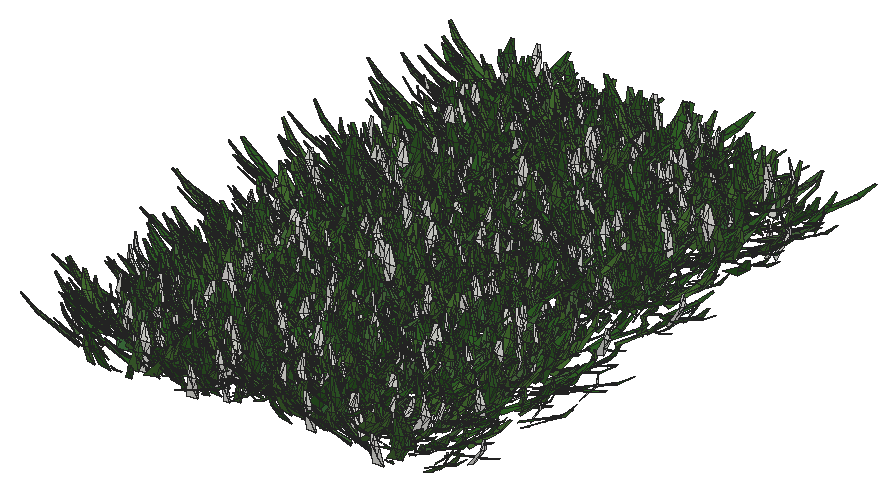
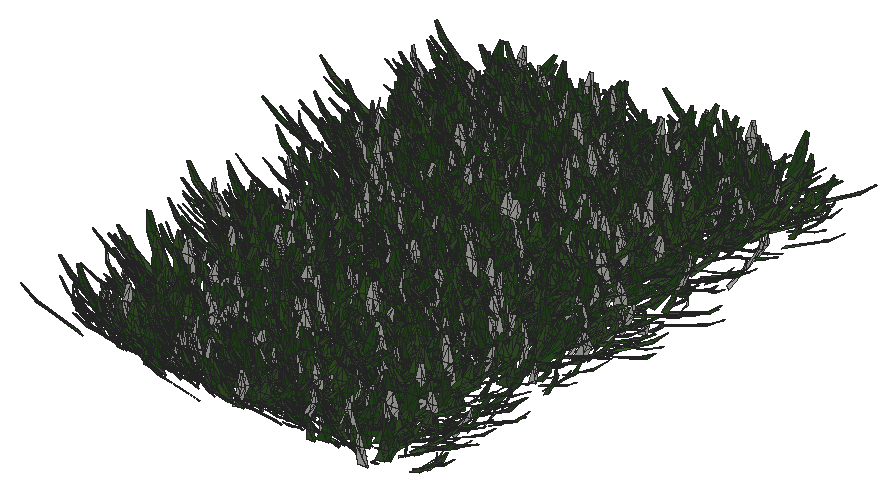
# SketchUp Ruby script. Lengths in inches.
U = 1.inch
M = Sketchup.active_model
def pt(a) = Geom::Point3d.new(a.map { |v| v * U })
def face(e, loops, mat)
  f = e.add_face(loops[0].map { |a| pt(a) })
  loops[1..].each { |l| e.add_face(l.map { |a| pt(a) }).erase! }
  f.material = f.back_material = mat if mat
  f
end
# faces: each face lists its corners as indices into pts; further lists are holes
def faces(e, pts, list, mat = nil) = list.each { |f| face(e, (f[0].is_a?(Array) ? f : [f]).map { |l| l.map { |i| pts[i] } }, mat) }
# xy, xz, yz: faces in a plane at the given z, y or x. An outline is a flat list of corners, or four numbers for a rectangle; further outlines are holes
def ring(l) = l.size == 4 ? [[l[0], l[1]], [l[2], l[1]], [l[2], l[3]], [l[0], l[3]]] : l.each_slice(2).to_a
def flat(e, list, mat, &to3) = list.each { |f| face(e, (f[0].is_a?(Array) ? f : [f]).map { |l| ring(l).map { |u, v| to3.(u, v) } }, mat) }
def xy(e, z, list, mat = nil) = flat(e, list, mat) { |x, y| [x, y, z] }
def xz(e, y, list, mat = nil) = flat(e, list, mat) { |x, z| [x, y, z] }
def yz(e, x, list, mat = nil) = flat(e, list, mat) { |y, z| [x, y, z] }
def lines(e, pts, list) = list.each { |a, b| e.add_line(pt(pts[a]), pt(pts[b])) }
# prism: a flat outline (further loops are holes) pulled along v
def prism(e, loops, v, mat = nil)
  f = face(e, loops, mat); d = Geom::Vector3d.new(v.map { |x| x * U })
  f.pushpull(f.normal.samedirection?(d) ? d.length : -d.length)
end
def box(e, o, s, mat = nil) = prism(e, [[o, [o[0] + s[0], o[1], o[2]], [o[0] + s[0], o[1] + s[1], o[2]], [o[0], o[1] + s[1], o[2]]]], [0, 0, s[2]], mat)
def at(x, y, z, deg = 0) = Geom::Transformation.translation(pt([x, y, z])) * Geom::Transformation.rotation(ORIGIN, Z_AXIS, deg.degrees)
def axes(o, x, y, z) = Geom::Transformation.new([*x, 0, *y, 0, *z, 0, *pt(o).to_a, 1])
def part(name) = M.definitions.add(name)
# library, detail: a bought-in or finely detailed component or shape, given as its bounding box
def library(name, o, s) = part(name).tap { |d| box(d.entities, o, s) }
def detail(e, o, s) = box(e.add_group.entities, o, s)
def put(e, d, t, mat = nil) = e.add_instance(d, t).tap { |i| i.material = mat if mat }
def group(e, t, mat = nil) = e.add_group.tap { |g| g.transformation = t; g.material = mat if mat }.entities
root = M.entities
M.materials.add("Material82").color = [68, 110, 58]
M.materials.add("Material83").color = [48, 90, 38]
M.materials.add("Material84").color = [68, 110, 48]
M.materials.add("Material85").color = [48, 90, 48]
M.materials.add("Material86").color = [58, 110, 58]
M.materials.add("Material87").color = [58, 90, 38]
M.materials.add("Material88").color = [68, 100, 58]
M.materials.add("Material89").color = [48, 100, 38]
c1 = part("grass00")
p = [[-0.6875,0.15,0],[-0.56,0.08,5.52],[-0.04,0.03,2.76],[0.48,-0.02,0],[0.35,-0.02,5.52],[-0.1,-0.14,5.52],
  [-0.12,0.65,8.37],[-0.42,0.65,8.37]]
faces(c1.entities,p,[[0,1,2,3],[3,2,4],[1,5,2],[5,4,2],[1,6,5],[4,5,6],[7,6,1]])
c2 = part("Group16\#1")
put(c2.entities,c1,axes([1.44,-0.61,-0.01],[0.05352,0.12609,0],[-0.10704,0.04543,0.07239],[0.06664,-0.02828,0.11628]),"Material85")
put(c2.entities,c1,axes([0.76,-0.15,-0.01],[0.04676,0.24062,0],[-0.23162,0.04501,0.06642],[0.0652,-0.01267,0.23595]),"Material82")
put(c2.entities,c1,axes([0.79,0.01,-0.01],[-0.00606,0.34651,0],[-0.34381,-0.00602,0.0432],[0.04319,0.00076,0.34386]))
put(c2.entities,c1,axes([1,0.23,-0.01],[-0.07192,0.31144,0],[-0.28722,-0.06632,0.1236],[0.12043,0.02781,0.29478]),"Material84")
put(c2.entities,c1,axes([1.66,0.77,-0.01],[-0.13828,0.29651,0],[-0.21551,-0.1005,0.22471],[0.20365,0.09498,0.23779]),"Material89")
put(c2.entities,c1,axes([0.6875,0.52,-0.01],[-0.18126,0.24051,0],[-0.22746,-0.17142,0.09788],[0.07817,0.05891,0.28481]),"Material84")
put(c2.entities,c1,axes([0.68,0.78,-0.01],[-0.215,0.18688,0],[-0.12385,-0.14248,0.21334],[0.13995,0.16101,0.18878]),"Material82")
put(c2.entities,c1,axes([0.56,1,-0.01],[-0.13756,0.07624,0],[-0.06159,-0.11112,0.0927],[0.04494,0.08108,0.12705]),"Material84")
put(c2.entities,c1,axes([0.2,0.64,-0.01],[-0.23729,0.07254,0],[-0.05711,-0.18681,0.153],[0.04473,0.14632,0.19535]),"Material89")
put(c2.entities,c1,axes([0.0625,0.72,-0.01],[-0.28874,0.02525,0],[-0.02179,-0.24916,0.14647],[0.01276,0.14591,0.25012]),"Material82")
put(c2.entities,c1,axes([-0.08,0.62,-0.01],[-0.34089,-0.04187,0],[0.03255,-0.26504,0.216],[-0.02633,0.21439,0.26703]),"Material89")
put(c2.entities,c1,axes([-0.34,0.98,-0.01],[-0.14314,-0.0493,0],[0.04397,-0.12769,0.06843],[-0.02228,0.0647,0.13505]),"Material89")
put(c2.entities,c1,axes([-0.87,1.45,-0.01],[-0.23488,-0.14114,0],[0.13761,-0.22901,0.06087],[-0.03135,0.05217,0.26717]))
put(c2.entities,c1,axes([-0.72,0.77,-0.01],[-0.14208,-0.13251,0],[0.07209,-0.0773,0.16301],[-0.11118,0.11922,0.1057]),"Material89")
put(c2.entities,c1,axes([-0.62,0.43,-0.01],[-0.14845,-0.21203,0],[0.18654,-0.13061,0.12304],[-0.10079,0.07057,0.22772]),"Material82")
put(c2.entities,c1,axes([-0.68,0.29,-0.01],[-0.13639,-0.32136,0],[0.31723,-0.13464,0.05579],[-0.05136,0.0218,0.34462]),"Material83")
put(c2.entities,c1,axes([-0.64,0.125,-0.01],[-0.0458,-0.23569,0],[0.22124,-0.043,0.08276],[-0.08124,0.01579,0.22538]),"Material86")
put(c2.entities,c1,axes([-1.6,-0.03,-0.01],[0.00576,-0.32897,0],[0.27526,0.00482,0.18018],[-0.18015,-0.00315,0.2753]),"Material84")
put(c2.entities,c1,axes([-1.36,-0.31,-0.01],[0.05718,-0.24765,0],[0.18172,0.04196,0.17267],[-0.16825,-0.03885,0.1865]),"Material89")
put(c2.entities,c1,axes([-1.54,-0.72,-0.01],[0.06537,-0.14017,0],[0.13555,0.06321,0.03939],[-0.0357,-0.01665,0.14956]))
put(c2.entities,c1,axes([-1.19,-0.9,-0.01],[0.09597,-0.12735,0],[0.11214,0.08451,0.07557],[-0.06035,-0.04548,0.14042]),"Material88")
put(c2.entities,c1,axes([-0.47,-0.54,-0.01],[0.11588,-0.10072,0],[0.0618,0.0711,0.12124],[-0.07953,-0.0915,0.0942]))
put(c2.entities,c1,axes([-0.47,-0.84,-0.01],[0.11927,-0.0661,0],[0.06603,0.11913,0.00646],[-0.00313,-0.00565,0.13621]),"Material84")
put(c2.entities,c1,axes([-0.38,-1.24,-0.01],[0.28037,-0.08571,0],[0.0618,0.20215,0.20315],[-0.05939,-0.19428,0.21139]),"Material88")
put(c2.entities,c1,axes([-0.06,-0.66,-0.01],[0.22719,-0.01987,0],[0.01247,0.14255,0.17758],[-0.01547,-0.17691,0.1431]),"Material87")
put(c2.entities,c1,axes([0.11,-0.89,-0.01],[0.14882,0.01828,0],[-0.01058,0.08611,0.12229],[0.01491,-0.12138,0.08676]),"Material85")
put(c2.entities,c1,axes([0.25,-0.72,-0.01],[0.20481,0.07053,0],[-0.06206,0.18022,0.10291],[0.03351,-0.0973,0.1906]),"Material85")
put(c2.entities,c1,axes([0.85,-1.42,-0.01],[0.16481,0.09904,0],[-0.09472,0.15762,0.05616],[0.02893,-0.04814,0.18389]),"Material84")
put(c2.entities,c1,axes([1.01,-1.09,-0.01],[0.21858,0.20385,0],[-0.17495,0.1876,0.15339],[0.10462,-0.11218,0.25652]),"Material89")
put(c2.entities,c1,axes([1.01,-0.71,-0.01],[0.08733,0.12473,0],[-0.06445,0.04512,0.13037],[0.1068,-0.07477,0.07867]),"Material85")
c3 = part("Group15\#1")
put(c3.entities,c2,at(0,0,0))
c4 = part("3darcstudiotree_grass00\#1")
put(c4.entities,c3,at(0,0,0))
put(root,c4,axes([777.29,306.87,-34.17],[1.677,-1.55355,0],[4.28787,0.71988,-0.03539],[0.14144,0.02375,1.51703]))
put(root,c4,axes([777.74,322.0625,-34.17],[-2.71685,-1.17622,0],[2.71806,-0.97644,-0.02128],[0.11147,-0.04005,1.95268]))
put(root,c4,axes([777.99,286.73,-34.17],[-3.01218,-1.1682,0],[2.32929,-0.93411,-0.00764],[0.03903,-0.01565,1.81511]))
put(root,c4,axes([778.03,333.52,-34.17],[0.25601,-1.60576,0],[3.7655,0.09337,-0.00515],[0.03185,0.00079,1.75106]))
put(root,c4,axes([777.02,340.01,-34.17],[3.21046,-0.42194,0],[1.31397,1.55496,-0.01535],[0.02427,0.02872,1.5577]))
put(root,c4,axes([777.04,312.04,-34.17],[-1.88352,1.24088,0],[-3.53635,-0.83485,-0.03562],[-0.13641,-0.0322,1.37892]))
put(root,c4,axes([777.76,283.93,-34.17],[0.35251,-1.39793,0],[3.51175,0.13773,-0.03727],[0.24286,0.00952,1.73202]))
put(root,c4,axes([778.03,289.67,-34.17],[-3.43821,0.20499,0],[-0.69374,-1.80975,-0.03474],[-0.02131,-0.0556,1.42794]))
put(root,c4,axes([777.09,298.68,-34.17],[-0.07716,1.61232,0],[-4.08051,-0.03037,-0.05443],[-0.27918,-0.00208,1.56933]))
put(root,c4,axes([778.64,320.22,-34.17],[1.28288,-1.22527,0],[4.05082,0.65965,-0.04448],[0.2416,0.03934,1.93016]))
put(root,c4,axes([778.91,328.61,-34.17],[-0.2981,-1.54731,0],[4.18924,-0.12553,-0.05563],[0.33136,-0.00993,1.88098]))
put(root,c4,axes([778.75,317.46,-34.17],[-0.54088,1.62044,0],[-3.31155,-0.17191,-0.03263],[-0.19335,-0.01004,1.49628]))
put(root,c4,axes([778.93,315.92,-34.17],[3.70566,-0.42814,0],[1.15173,1.5504,-0.01036],[0.01836,0.02471,1.93559]))
put(root,c4,axes([779.4375,281.24,-34.17],[2.92691,-1.3802,0],[3.11862,1.02859,-0.02296],[0.10607,0.03499,1.8355]))
put(root,c4,axes([780,338.09,-34.17],[-3.14741,0.41412,0],[-1.12782,-1.33315,-0.01591],[-0.02767,-0.03271,1.46774]))
put(root,c4,axes([779.23,335.22,-34.17],[-0.97344,1.33602,0],[-4.5066,-0.51069,-0.06106],[-0.24596,-0.02787,1.47293]))
put(root,c4,axes([779.06,304.44,-34.17],[4.64499,-0.27977,0],[0.53132,1.372,-0.02943],[0.02555,0.06597,1.51666]))
put(root,c4,axes([780.51,302.05,-34.17],[-0.18207,-1.50592,0],[4.09357,-0.07698,-0.05646],[0.28834,-0.00542,1.57058]))
put(root,c4,axes([779.18,291.67,-34.17],[2.47814,1.17598,0],[-3.14029,1.02922,-0.05468],[-0.21842,0.07159,1.58958]))
put(root,c4,axes([779.15,313.96,-34.17],[4.42055,0.62646,0],[-1.4719,1.61538,-0.03831],[-0.06085,0.06679,1.53223]))
put(root,c4,axes([779.68,330.81,-34.17],[4.51641,-0.1704,0],[0.33815,1.39393,-0.00501],[0.00291,0.012,1.62495]))
put(root,c4,axes([779.375,293.85,-34.17],[2.33395,1.59128,0],[-3.69314,0.84246,-0.02506],[-0.12399,0.02828,1.82822]))
put(root,c4,axes([779.96,285.62,-34.17],[3.72841,-0.11021,0],[0.34874,1.83494,-0.00347],[0.00143,0.00753,1.92949]))
put(root,c4,axes([780.95,326.92,-34.17],[-2.15234,1.14546,0],[-3.3995,-0.99347,-0.05517],[-0.2418,-0.07066,1.72999]))
put(root,c4,axes([780.26,300.64,-34.17],[2.3917,1.38211,0],[-2.775,0.74686,-0.01403],[-0.09111,0.02452,1.97952]))
put(root,c4,axes([780.35,309.31,-34.17],[3.05644,0.96272,0],[-2.54771,1.25799,-0.04015],[-0.1144,0.05649,1.39698]))
put(root,c4,axes([780.91,296.33,-34.17],[0.44258,1.4547,0],[-3.4051,0.16112,-0.01784],[-0.12417,0.00588,1.80168]))
put(root,c4,axes([782.55,323.88,-34.17],[-1.45799,-1.43911,0],[3.11235,-0.49041,-0.01431],[0.09188,-0.01448,1.73701]))
put(root,c4,axes([782.7,283.47,-34.17],[-2.77273,1.25915,0],[-2.61353,-0.89509,-0.01448],[-0.05898,-0.0202,1.39954]))
put(root,c4,axes([783.67,285,-34.17],[-3.67224,-0.62774,0],[1.3268,-1.20717,-0.04544],[0.10775,-0.09803,1.4908]))
put(root,c4,axes([783.92,317.6,-34.17],[-4.47177,0.4092,0],[-0.80597,-1.36984,-0.03599],[-0.04373,-0.07433,1.43677]))
put(root,c4,axes([783.3,295.9,-34.17],[-3.07968,1.30519,0],[-3.32937,-1.22181,-0.01383],[-0.04412,-0.01619,1.48532]))
put(root,c4,axes([784.08,339.19,-34.17],[-3.54635,0.32604,0],[-1.06041,-1.79388,-0.06463],[-0.05576,-0.09432,1.33032]))
put(root,c4,axes([782.85,307.32,-34.17],[3.91717,0.58785,0],[-1.40512,1.45623,-0.01203],[-0.02325,0.0241,1.60927]))
put(root,c4,axes([784.71,302.46,-34.17],[-1.04981,-1.26066,0],[3.51989,-0.45588,-0.02104],[0.10484,-0.01358,1.45661]))
put(root,c4,axes([783.97,299.02,-34.17],[3.15172,-0.92963,0],[2.70365,1.42561,-0.02614],[0.06865,0.0362,1.48366]))
put(root,c4,axes([784.75,305.26,-34.17],[-4.56421,0.17831,0],[-0.33265,-1.32435,-0.0174],[-0.0117,-0.04658,1.72585]))
put(root,c4,axes([785.23,330.95,-34.17],[-3.08784,-0.53374,0],[1.78756,-1.6084,-0.00176],[0.00414,-0.00372,1.95594]))
put(root,c4,axes([784.29,291.37,-34.17],[-2.14552,1.35971,0],[-3.80804,-0.93454,-0.04897],[-0.2422,-0.05944,1.9584]))
put(root,c4,axes([783.75,288.08,-34.17],[3.03533,0.518,0],[-1.31858,1.2017,-0.02703],[-0.08286,0.07551,1.9211]))
put(root,c4,axes([785.59,313.28,-34.17],[-2.79081,-0.68685,0],[2.20267,-1.39196,-0.00523],[0.01654,-0.01045,1.86317]))
put(root,c4,axes([785.72,316.69,-34.17],[-3.42781,-0.73376,0],[1.91044,-1.38806,-0.04387],[0.11882,-0.08633,1.70431]))
put(root,c4,axes([785.03,289.42,-34.17],[-3.41152,0.77464,0],[-2.34689,-1.60751,-0.0199],[-0.0471,-0.03226,1.67187]))
put(root,c4,axes([784.04,312.07,-34.17],[1.53269,1.16919,0],[-3.90157,0.79546,-0.03477],[-0.15934,0.03249,1.69826]))
put(root,c4,axes([785.32,300.03,-34.17],[-2.82754,1.11661,0],[-2.90837,-1.14544,-0.05526],[-0.21558,-0.0849,1.69871]))
put(root,c4,axes([785.34,293.44,-34.17],[2.39859,-1.38317,0],[2.89597,0.78107,-0.02882],[0.1286,0.03468,1.42183]))
put(root,c4,axes([785.76,337.85,-34.17],[0.37671,-1.60669,0],[3.58296,0.13066,-0.04487],[0.23434,0.00855,1.41449]))
put(root,c4,axes([786.17,336.35,-34.17],[-4.41181,-0.09171,0],[0.23476,-1.75641,-0.0488],[0.01273,-0.09527,1.65721]))
put(root,c4,axes([786.03,281.67,-34.17],[-3.47293,0.19496,0],[-0.50842,-1.40863,-0.03826],[-0.03299,-0.09141,1.65468]))
put(root,c4,axes([786.59,332.71,-34.17],[-4.2727,-0.29638,0],[0.78575,-1.76178,-0.04722],[0.03378,-0.07573,1.40384]))
put(root,c4,axes([785.25,328.23,-34.17],[-0.9668,1.66725,0],[-3.92404,-0.3539,-0.0233],[-0.11915,-0.01075,1.58282]))
put(root,c4,axes([785.3,309.55,-34.17],[3.78841,0.96012,0],[-2.55963,1.5708,-0.03131],[-0.07104,0.04359,1.48921]))
put(root,c4,axes([785.54,322.55,-34.17],[2.7139,1.45109,0],[-3.63417,1.0571,-0.05484],[-0.17137,0.04985,1.31443]))
put(root,c4,axes([786.1,320.54,-34.17],[3.41186,0.04199,0],[-0.11049,1.39641,-0.01718],[-0.0038,0.04797,1.88076]))
put(root,c4,axes([788.18,299.01,-34.17],[-3.09292,-0.92086,0],[2.57207,-1.3436,-0.01411],[0.04505,-0.02353,1.69584]))
put(root,c4,axes([786.33,326.3125,-34.17],[0.1551,1.54916,0],[-4.73746,0.07377,-0.04149],[-0.18002,0.0028,1.54325]))
put(root,c4,axes([788.36,317.79,-34.17],[0.67498,-1.80639,0],[4.18251,0.24307,-0.00777],[0.03281,0.00191,1.3523]))
put(root,c4,axes([788.52,313.77,-34.17],[-0.75947,-1.30953,0],[4.19896,-0.37875,-0.04627],[0.26037,-0.02349,1.86363]))
put(root,c4,axes([788.5625,300.08,-34.17],[-4.1346,0.13575,0],[-0.2838,-1.34436,-0.02559],[-0.01617,-0.0766,1.95328]))
put(root,c4,axes([789.34,311.39,-34.17],[1.00092,-1.32759,0],[4.42574,0.51896,-0.06029],[0.29852,0.035,1.78762]))
put(root,c4,axes([789.04,332.57,-34.17],[2.10537,-1.23806,0],[3.71835,0.98344,-0.05795],[0.27877,0.07373,1.94389]))
put(root,c4,axes([788.38,287.45,-34.17],[3.79547,0.16316,0],[-0.37027,1.33962,-0.03498],[-0.02197,0.07948,1.48455]))
put(root,c4,axes([789.23,306.96,-34.17],[-3.00276,0.99555,0],[-2.11915,-0.9941,-0.00081],[-0.00373,-0.00175,1.76997]))
put(root,c4,axes([790.35,325.16,-34.17],[-0.04764,-1.42757,0],[4.50476,-0.02338,-0.00745],[0.04284,-0.00022,1.94284]))
put(root,c4,axes([789.05,283.19,-34.17],[0.27257,1.5962,0],[-3.57048,0.09483,-0.04154],[-0.28788,0.00765,1.86323]))
put(root,c4,axes([790.49,320.39,-34.17],[-4.51182,-0.35471,0],[0.87439,-1.72977,-0.01918],[0.02129,-0.04212,1.90358]))
put(root,c4,axes([789.26,327.35,-34.17],[2.9902,-0.77103,0],[1.83544,1.10708,-0.045],[0.13449,0.08112,1.37282]))
put(root,c4,axes([790.54,305.3,-34.17],[0.52861,-1.48035,0],[4.44113,0.24665,-0.00524],[0.03043,0.00169,1.97007]))
put(root,c4,axes([788.83,294.74,-34.17],[1.62026,1.14881,0],[-2.90984,0.63829,-0.00131],[-0.00892,0.00196,1.9458]))
put(root,c4,axes([789.86,285.1875,-34.17],[-3.07094,0.93295,0],[-2.23562,-1.14452,-0.00087],[-0.00325,-0.00166,1.68429]))
put(root,c4,axes([790.9,291.54,-34.17],[-1.32818,-1.26932,0],[4.11875,-0.67029,-0.01762],[0.07227,-0.01176,1.48208]))
put(root,c4,axes([789,289.16,-34.17],[3.48613,0.95688,0],[-2.23612,1.26704,-0.01513],[-0.04219,0.02391,1.43215]))
put(root,c4,axes([790.08,322.25,-34.17],[3.73229,-0.67208,0],[1.78653,1.54305,-0.05401],[0.10032,0.08665,1.44188]))
put(root,c4,axes([791.73,335.35,-34.17],[-3.64932,-0.7532,0],[1.94147,-1.463,-0.05348],[0.14522,-0.10943,1.83786]))
put(root,c4,axes([790.43,309.52,-34.17],[4.39358,-0.14103,0],[0.35283,1.70956,-0.02372],[0.00876,0.04243,1.48337]))
put(root,c4,axes([791.92,336.93,-34.17],[-4.22243,0.41861,0],[-0.86072,-1.35028,-0.03206],[-0.04838,-0.0759,1.63785]))
put(root,c4,axes([790.9375,328.72,-34.17],[2.4549,0.99675,0],[-3.14112,1.20322,-0.03466],[-0.14383,0.05509,1.89896]))
put(root,c4,axes([790.98,315.6,-34.17],[3.48474,0.89145,0],[-2.45497,1.49256,-0.05832],[-0.13986,0.08503,1.48992]))
put(root,c4,axes([791.51,331.39,-34.17],[-0.03901,1.43427,0],[-3.74587,-0.01585,-0.03184],[-0.19446,-0.00082,1.71482]))
put(root,c4,axes([791.9,303.07,-34.17],[-1.95042,1.47202,0],[-4.16072,-0.85742,-0.06253],[-0.2988,-0.06158,1.89715]))
put(root,c4,axes([791.8,296.46,-34.17],[3.54296,-0.10072,0],[0.24357,1.33252,-0.00836],[0.00467,0.02557,1.97523]))
put(root,c4,axes([794,313.82,-34.17],[-3.58618,-0.76762,0],[2.12856,-1.54662,-0.04044],[0.10752,-0.07813,1.86421]))
put(root,c4,axes([792.02,339.32,-34.17],[3.38325,1.26435,0],[-2.73925,1.14001,-0.00751],[-0.0314,0.01307,1.8142]))
put(root,c4,axes([794.27,309.27,-34.17],[-3.71376,-0.4791,0],[1.06109,-1.27925,-0.035],[0.07367,-0.08882,1.73222]))
put(root,c4,axes([794.82,329.42,-34.17],[-3.76687,-0.82913,0],[2.27178,-1.60524,-0.0179],[0.04066,-0.02873,1.62858]))
put(root,c4,axes([793.99,291.75,-34.17],[-3.28554,0.84585,0],[-2.43757,-1.4726,-0.04574],[-0.1384,-0.08361,1.85022]))
put(root,c4,axes([794.73,290.41,-34.17],[0.43132,-1.66774,0],[3.95027,0.1589,-0.00761],[0.04938,0.00199,1.94156]))
put(root,c4,axes([794.99,317.49,-34.17],[-3.03865,-1.23581,0],[2.76731,-1.05827,-0.04714],[0.18592,-0.0711,1.58733]))
put(root,c4,axes([793.58,286.78,-34.17],[4.71636,-0.1967,0],[0.48906,1.82382,-0.02611],[0.01545,0.05763,1.96192]))
put(root,c4,axes([794.67,320.03,-34.17],[-3.07129,1.23004,0],[-2.90171,-1.12685,-0.02428],[-0.07533,-0.02925,1.32917]))
put(root,c4,axes([795.58,294.77,-34.17],[-3.14124,-0.52931,0],[1.80451,-1.66556,-0.04539],[0.09971,-0.09203,1.92461]))
put(root,c4,axes([794.3,338.31,-34.17],[4.37264,-0.16186,0],[0.38997,1.63854,-0.03728],[0.02119,0.08905,1.90298]))
put(root,c4,axes([794.65,332.74,-34.17],[4.22982,-0.69798,0],[1.45654,1.37281,-0.04818],[0.09708,0.0915,1.47658]))
put(root,c4,axes([794.91,331.78,-34.17],[3.5272,-0.10967,0],[0.36977,1.84972,-0.03935],[0.01267,0.0634,1.44542]))
put(root,c4,axes([795.64,324.05,-34.17],[2.22522,-0.98382,0],[3.26699,1.14926,-0.04874],[0.15967,0.05617,1.44038]))
put(root,c4,axes([794.85,298.49,-34.17],[4.40761,-0.00182,0],[0.00468,1.76466,-0.04894],[0.00022,0.08123,1.41164]))
put(root,c4,axes([795.02,339.18,-34.17],[3.37216,0.16863,0],[-0.47809,1.48691,-0.01144],[-0.0086,0.02673,1.7012]))
put(root,c4,axes([796.74,316.68,-34.17],[-3.1255,-0.93872,0],[2.35839,-1.22127,-0.01582],[0.04515,-0.02338,1.37394]))
put(root,c4,axes([795.69,312.24,-34.17],[-2.15998,1.50569,0],[-3.5128,-0.78375,-0.02589],[-0.10439,-0.02329,1.40149]))
put(root,c4,axes([796.18,335.6,-34.17],[2.50422,-1.12718,0],[2.64209,0.91293,-0.00209],[0.0092,0.00318,1.54397]))
put(root,c4,axes([796.33,327.24,-34.17],[-3.79899,1.04858,0],[-2.13311,-1.20197,-0.01309],[-0.05055,-0.02848,1.87779]))
put(root,c4,axes([797,297.02,-34.17],[-0.77442,-1.59147,0],[3.42237,-0.25901,-0.00431],[0.02185,-0.00165,1.34772]))
put(root,c4,axes([797.28,283.77,-34.17],[-1.56215,-1.16443,0],[3.47638,-0.72535,-0.0302],[0.1517,-0.03165,1.67548]))
put(root,c4,axes([797.36,302.51,-34.17],[0.16922,-1.40325,0],[3.56749,0.06691,-0.0123],[0.08099,0.00152,1.7643]))
put(root,c4,axes([796.1875,306.82,-34.17],[3.21803,0.34517,0],[-1.06694,1.54707,-0.02379],[-0.03071,0.04453,1.49895]))
put(root,c4,axes([795.95,300.53,-34.17],[1.18275,1.22871,0],[-4.35683,0.65227,-0.02635],[-0.11985,0.01794,1.69955]))
put(root,c4,axes([797.61,322.41,-34.17],[-4.55654,0.30056,0],[-0.72952,-1.72007,-0.00717],[-0.00538,-0.01268,1.50735]))
put(root,c4,axes([797.1,305.49,-34.17],[2.66801,-0.76193,0],[2.24823,1.2244,-0.04376],[0.15596,0.08494,1.7457]))
put(root,c4,axes([799.2,313.06,-34.17],[-2.4386,-1.43306,0],[3.07254,-0.81318,-0.00883],[0.05033,-0.01332,1.90461]))
put(root,c4,axes([799.57,331.49,-34.17],[-2.69612,-1.17454,0],[3.29179,-1.17522,-0.01753],[0.05781,-0.02064,1.48083]))
put(root,c4,axes([797.53,285.37,-34.17],[-0.169,1.77802,0],[-4.32571,-0.06395,-0.00219],[-0.00941,-0.00014,1.39308]))
put(root,c4,axes([799.77,289.02,-34.17],[-3.83813,-1.06248,0],[2.06139,-1.15817,-0.02484],[0.08815,-0.04953,1.66133]))
put(root,c4,axes([799.46,325.34,-34.17],[-4.08007,0.11151,0],[-0.22831,-1.29918,-0.01842],[-0.00694,-0.03947,1.34789]))
put(root,c4,axes([799.94,283.58,-34.17],[-3.13096,0.65051,0],[-1.62991,-1.22011,-0.01732],[-0.0588,-0.04402,1.90951]))
put(root,c4,axes([801.15,335.92,-34.17],[-1.34356,-1.54381,0],[4.22745,-0.57221,-0.00214],[0.01038,-0.00141,1.72072]))
put(root,c4,axes([799.21,291.125,-34.17],[3.83567,0.80348,0],[-1.71741,1.27513,-0.04207],[-0.13622,0.10114,1.89419]))
put(root,c4,axes([799.63,307.22,-34.17],[2.14752,1.24419,0],[-2.84206,0.76295,-0.02533],[-0.12904,0.03464,1.58831]))
put(root,c4,axes([800.24,329.55,-34.17],[4.00755,-0.76372,0],[1.77132,1.44561,-0.00312],[0.00773,0.00631,1.73901]))
put(root,c4,axes([799.93,300.73,-34.17],[0.92286,1.78615,0],[-4.03148,0.32396,-0.0503],[-0.25163,0.02022,1.57458]))
put(root,c4,axes([800.27,315.79,-34.17],[-1.5079,1.48015,0],[-3.78766,-0.60014,-0.02547],[-0.10708,-0.01697,1.38631]))
put(root,c4,axes([801.32,297.77,-34.17],[0.88426,-1.72062,0],[4.38154,0.35021,-0.041],[0.21175,0.01693,1.76588]))
put(root,c4,axes([800.14,293.66,-34.17],[4.1439,0.48612,0],[-1.21296,1.60815,-0.03162],[-0.038,0.05038,1.3441]))
put(root,c4,axes([800,308.79,-34.17],[2.12924,1.06786,0],[-3.55371,1.10206,-0.01217],[-0.05143,0.01595,1.82194]))
put(root,c4,axes([801.57,284.69,-34.17],[1.5808,-1.43275,0],[3.65536,0.62726,-0.04597],[0.19603,0.03364,1.38947]))
put(root,c4,axes([802.46,288,-34.17],[-4.27451,-0.64112,0],[1.27307,-1.32012,-0.04106],[0.09351,-0.09696,1.71966]))
put(root,c4,axes([802.38,332.92,-34.17],[-3.75297,0.08152,0],[-0.23562,-1.68719,-0.02509],[-0.00578,-0.04142,1.34616]))
put(root,c4,axes([802.375,338.3,-34.17],[-3.08585,0.75112,0],[-1.75968,-1.12437,-0.03387],[-0.09597,-0.06132,1.3548]))
put(root,c4,axes([803.03,323.26,-34.17],[-0.74737,-1.75822,0],[4.00395,-0.2647,-0.02808],[0.1526,-0.01009,1.67665]))
put(root,c4,axes([802.27,304.49,-34.17],[2.37533,-1.57622,0],[3.03149,0.71052,-0.0411],[0.20378,0.04776,1.52451]))
put(root,c4,axes([801.47,317.97,-34.17],[3.22242,0.46316,0],[-1.61234,1.7447,-0.03532],[-0.06153,0.06658,1.79519]))
put(root,c4,axes([801.96,312.34,-34.17],[0.53134,1.4221,0],[-3.42638,0.19911,-0.04131],[-0.21204,0.01232,1.34689]))
put(root,c4,axes([802.45,303.55,-34.17],[3.9417,-1.03975,0],[1.84996,1.09076,-0.03191],[0.12762,0.07525,1.79443]))
put(root,c4,axes([802.83,296.27,-34.17],[3.56947,-0.45549,0],[1.31887,1.60745,-0.01717],[0.02449,0.02985,1.48777]))
put(root,c4,axes([802.91,319.66,-34.17],[0.55525,1.71346,0],[-3.482,0.17549,-0.04145],[-0.30813,0.01553,1.97198]))
put(root,c4,axes([802.66,326.65,-34.17],[3.66484,0.89609,0],[-2.00603,1.27601,-0.03504],[-0.12347,0.07854,1.90819]))
put(root,c4,axes([804.875,289.59,-34.17],[-1.10349,-1.4395,0],[4.41957,-0.52692,-0.03772],[0.14279,-0.01702,1.36861]))
put(root,c4,axes([804.67,319.5,-34.17],[-2.20687,1.14075,0],[-3.09016,-0.92978,-0.05103],[-0.23957,-0.07208,1.72023]))
put(root,c4,axes([805.13,331.53,-34.17],[-3.32366,1.12138,0],[-2.70082,-1.24501,-0.05065],[-0.15287,-0.07047,1.44592]))
put(root,c4,axes([806.22,316.28,-34.17],[-2.7638,-1.30283,0],[3.13183,-1.03331,-0.01878],[0.07913,-0.02611,1.68146]))
put(root,c4,axes([806.45,309,-34.17],[-3.16827,-0.67396,0],[1.62868,-1.19079,-0.04409],[0.1208,-0.08832,1.48398]))
put(root,c4,axes([806.2,317.34,-34.17],[-4.1698,0.79339,0],[-1.666,-1.36181,-0.02532],[-0.06287,-0.05139,1.64221]))
put(root,c4,axes([805.17,337.66,-34.17],[3.81533,0.48086,0],[-1.13696,1.40304,-0.03842],[-0.0798,0.09848,1.90991]))
put(root,c4,axes([805.77,302.06,-34.17],[3.77642,-0.7823,0],[1.66108,1.24712,-0.02304],[0.07142,0.05362,1.78453]))
put(root,c4,axes([807.3,329.27,-34.17],[0.63263,-1.77026,0],[4.09912,0.22783,-0.02402],[0.14113,0.00784,1.84088]))
put(root,c4,axes([807.44,293.54,-34.17],[-4.44839,0.03138,0],[-0.07411,-1.6342,-0.01042],[-0.00109,-0.02408,1.82123]))
put(root,c4,axes([807.43,282.67,-34.17],[-3.4085,0.44598,0],[-1.18576,-1.40948,-0.04681],[-0.08042,-0.0956,1.53984]))
put(root,c4,axes([806.18,292.31,-34.17],[3.54482,0.3991,0],[-1.20365,1.66273,-0.00872],[-0.01104,0.01525,1.51538]))
put(root,c4,axes([806.8125,322.3,-34.17],[-0.28998,1.73456,0],[-3.34694,-0.08702,-0.03816],[-0.29536,-0.00768,1.95014]))
put(root,c4,axes([806.03,287.11,-34.17],[3.41397,1.21641,0],[-2.3032,1.00536,-0.00582],[-0.0237,0.01035,1.56404]))
put(root,c4,axes([806.16,298.54,-34.17],[2.93721,1.2592,0],[-3.10849,1.12772,-0.033],[-0.144,0.05224,1.87715]))
put(root,c4,axes([808.32,300.11,-34.17],[-1.1478,-1.40641,0],[4.093,-0.51953,-0.0477],[0.19511,-0.02477,1.385]))
put(root,c4,axes([808.71,285.97,-34.17],[-2.49924,-1.08664,0],[2.82442,-1.01033,-0.0539],[0.19999,-0.07154,1.43163]))
put(root,c4,axes([807.1,305.5,-34.17],[2.93445,0.88211,0],[-2.13254,1.10335,-0.01463],[-0.05848,0.03025,1.73802]))
put(root,c4,axes([807.22,297,-34.17],[3.48566,0.55514,0],[-1.55719,1.52067,-0.03343],[-0.07577,0.07399,1.88641]))
put(root,c4,axes([807.68,335.54,-34.17],[-0.15322,1.4871,0],[-3.57108,-0.05722,-0.03031],[-0.19833,-0.00318,1.75443]))
put(root,c4,axes([807.38,314.39,-34.17],[3.31433,0.47754,0],[-1.51472,1.63504,-0.04863],[-0.07862,0.08486,1.5585]))
